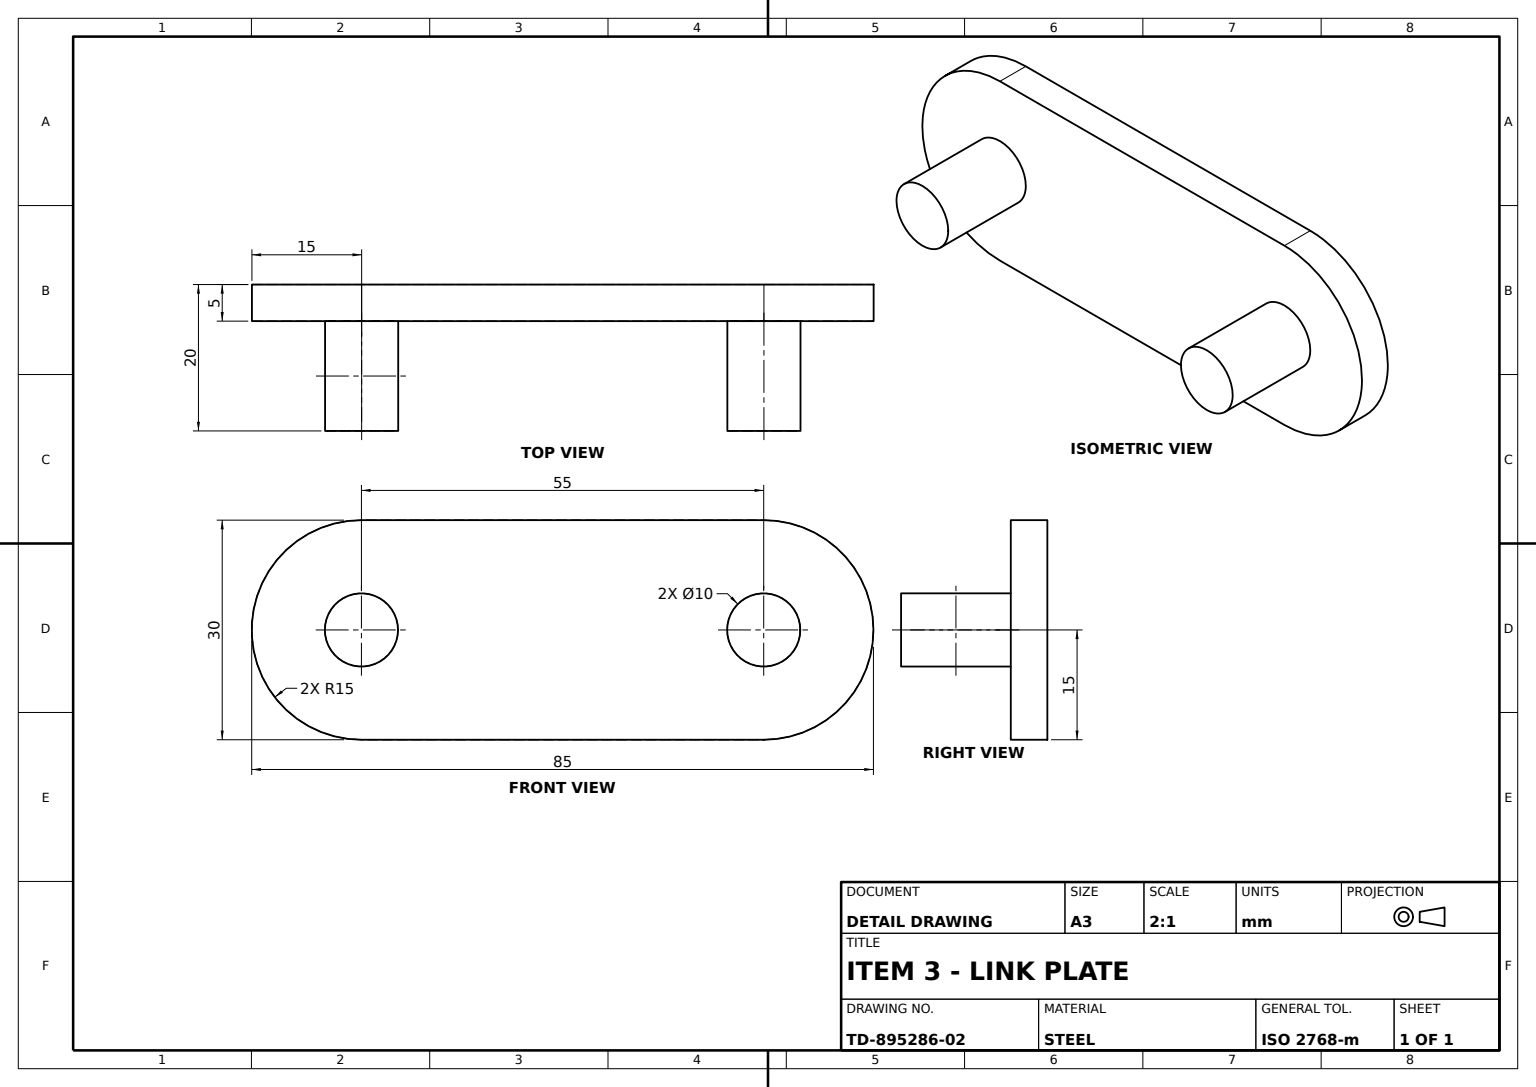
ISO-10303-21;
HEADER;
FILE_DESCRIPTION((''),'2;1');
FILE_NAME('','',(''),(''),'','','');
FILE_SCHEMA(('AUTOMOTIVE_DESIGN'));
ENDSEC;
DATA;
#1=APPLICATION_CONTEXT('');
#2=PRODUCT_CONTEXT('',#1,'mechanical');
#3=PRODUCT('','','',(#2));
#4=PRODUCT_DEFINITION_FORMATION('','',#3);
#5=PRODUCT_DEFINITION_CONTEXT('',#1,'design');
#6=PRODUCT_DEFINITION('','',#4,#5);
#7=PRODUCT_DEFINITION_SHAPE('','',#6);
#8=(LENGTH_UNIT()NAMED_UNIT(*)SI_UNIT(.MILLI.,.METRE.));
#9=(NAMED_UNIT(*)PLANE_ANGLE_UNIT()SI_UNIT($,.RADIAN.));
#10=(NAMED_UNIT(*)SI_UNIT($,.STERADIAN.)SOLID_ANGLE_UNIT());
#11=UNCERTAINTY_MEASURE_WITH_UNIT(LENGTH_MEASURE(1.E-05),#8,'distance_accuracy_value','');
#12=(GEOMETRIC_REPRESENTATION_CONTEXT(3)GLOBAL_UNCERTAINTY_ASSIGNED_CONTEXT((#11))GLOBAL_UNIT_ASSIGNED_CONTEXT((#8,#9,#10))REPRESENTATION_CONTEXT('',''));
#13=CARTESIAN_POINT('',(-22.5,0.,0.));
#14=VERTEX_POINT('',#13);
#15=CARTESIAN_POINT('',(-32.5,0.,0.));
#16=VERTEX_POINT('',#15);
#17=CARTESIAN_POINT('',(-27.5,0.,0.));
#18=DIRECTION('',(0.,0.,1.));
#19=DIRECTION('',(1.,0.,0.));
#20=AXIS2_PLACEMENT_3D('',#17,#18,#19);
#21=CIRCLE('',#20,5.);
#22=EDGE_CURVE('',#14,#16,#21,.T.);
#23=ORIENTED_EDGE('',*,*,#22,.T.);
#24=CARTESIAN_POINT('',(-32.5,0.,15.));
#25=VERTEX_POINT('',#24);
#26=DIRECTION('',(0.,0.,-1.));
#27=VECTOR('',#26,1000.);
#28=LINE('',#24,#27);
#29=EDGE_CURVE('',#25,#16,#28,.T.);
#30=ORIENTED_EDGE('',*,*,#29,.F.);
#31=CARTESIAN_POINT('',(-22.5,0.,15.));
#32=VERTEX_POINT('',#31);
#33=CARTESIAN_POINT('',(-27.5,0.,15.));
#34=AXIS2_PLACEMENT_3D('',#33,#18,#19);
#35=CIRCLE('',#34,5.);
#36=EDGE_CURVE('',#32,#25,#35,.T.);
#37=ORIENTED_EDGE('',*,*,#36,.F.);
#38=LINE('',#31,#27);
#39=EDGE_CURVE('',#32,#14,#38,.T.);
#40=ORIENTED_EDGE('',*,*,#39,.T.);
#41=EDGE_LOOP('',(#23,#30,#37,#40));
#42=FACE_OUTER_BOUND('',#41,.T.);
#43=DIRECTION('',(-1.,0.,0.));
#44=AXIS2_PLACEMENT_3D('',#33,#26,#43);
#45=CYLINDRICAL_SURFACE('',#44,5.);
#46=ADVANCED_FACE('',(#42),#45,.T.);
#47=EDGE_CURVE('',#16,#14,#21,.T.);
#48=ORIENTED_EDGE('',*,*,#47,.T.);
#49=ORIENTED_EDGE('',*,*,#39,.F.);
#50=EDGE_CURVE('',#25,#32,#35,.T.);
#51=ORIENTED_EDGE('',*,*,#50,.F.);
#52=ORIENTED_EDGE('',*,*,#29,.T.);
#53=EDGE_LOOP('',(#48,#49,#51,#52));
#54=FACE_OUTER_BOUND('',#53,.T.);
#55=ADVANCED_FACE('',(#54),#45,.T.);
#56=CARTESIAN_POINT('',(27.5,15.,-5.));
#57=VERTEX_POINT('',#56);
#58=CARTESIAN_POINT('',(27.5,15.,0.));
#59=VERTEX_POINT('',#58);
#60=VECTOR('',#18,1000.);
#61=LINE('',#56,#60);
#62=EDGE_CURVE('',#57,#59,#61,.T.);
#63=ORIENTED_EDGE('',*,*,#62,.F.);
#64=CARTESIAN_POINT('',(-27.5,15.,-5.));
#65=VERTEX_POINT('',#64);
#66=VECTOR('',#43,1000.);
#67=LINE('',#56,#66);
#68=EDGE_CURVE('',#57,#65,#67,.T.);
#69=ORIENTED_EDGE('',*,*,#68,.T.);
#70=CARTESIAN_POINT('',(-27.5,15.,0.));
#71=VERTEX_POINT('',#70);
#72=LINE('',#64,#60);
#73=EDGE_CURVE('',#65,#71,#72,.T.);
#74=ORIENTED_EDGE('',*,*,#73,.T.);
#75=LINE('',#58,#66);
#76=EDGE_CURVE('',#59,#71,#75,.T.);
#77=ORIENTED_EDGE('',*,*,#76,.F.);
#78=EDGE_LOOP('',(#63,#69,#74,#77));
#79=FACE_OUTER_BOUND('',#78,.T.);
#80=DIRECTION('',(0.,1.,0.));
#81=AXIS2_PLACEMENT_3D('',#56,#80,#43);
#82=PLANE('',#81);
#83=ADVANCED_FACE('',(#79),#82,.T.);
#84=CARTESIAN_POINT('',(32.5,0.,15.));
#85=VERTEX_POINT('',#84);
#86=CARTESIAN_POINT('',(22.5,0.,15.));
#87=VERTEX_POINT('',#86);
#88=CARTESIAN_POINT('',(27.5,0.,15.));
#89=AXIS2_PLACEMENT_3D('',#88,#18,#19);
#90=CIRCLE('',#89,5.);
#91=EDGE_CURVE('',#85,#87,#90,.T.);
#92=ORIENTED_EDGE('',*,*,#91,.T.);
#93=EDGE_CURVE('',#87,#85,#90,.T.);
#94=ORIENTED_EDGE('',*,*,#93,.T.);
#95=EDGE_LOOP('',(#92,#94));
#96=FACE_OUTER_BOUND('',#95,.T.);
#97=CARTESIAN_POINT('',(0.,0.,15.));
#98=AXIS2_PLACEMENT_3D('',#97,#18,#19);
#99=PLANE('',#98);
#100=ADVANCED_FACE('',(#96),#99,.T.);
#101=CARTESIAN_POINT('',(-27.5,-15.,-5.));
#102=VERTEX_POINT('',#101);
#103=CARTESIAN_POINT('',(-27.5,0.,-5.));
#104=AXIS2_PLACEMENT_3D('',#103,#18,#19);
#105=CIRCLE('',#104,15.);
#106=EDGE_CURVE('',#65,#102,#105,.T.);
#107=ORIENTED_EDGE('',*,*,#106,.T.);
#108=CARTESIAN_POINT('',(-27.5,-15.,0.));
#109=VERTEX_POINT('',#108);
#110=LINE('',#101,#60);
#111=EDGE_CURVE('',#102,#109,#110,.T.);
#112=ORIENTED_EDGE('',*,*,#111,.T.);
#113=CIRCLE('',#20,15.);
#114=EDGE_CURVE('',#71,#109,#113,.T.);
#115=ORIENTED_EDGE('',*,*,#114,.F.);
#116=ORIENTED_EDGE('',*,*,#73,.F.);
#117=EDGE_LOOP('',(#107,#112,#115,#116));
#118=FACE_OUTER_BOUND('',#117,.T.);
#119=CYLINDRICAL_SURFACE('',#104,15.);
#120=ADVANCED_FACE('',(#118),#119,.T.);
#121=ORIENTED_EDGE('',*,*,#91,.F.);
#122=CARTESIAN_POINT('',(32.5,0.,0.));
#123=VERTEX_POINT('',#122);
#124=LINE('',#84,#27);
#125=EDGE_CURVE('',#85,#123,#124,.T.);
#126=ORIENTED_EDGE('',*,*,#125,.T.);
#127=CARTESIAN_POINT('',(22.5,0.,0.));
#128=VERTEX_POINT('',#127);
#129=CARTESIAN_POINT('',(27.5,0.,0.));
#130=AXIS2_PLACEMENT_3D('',#129,#18,#19);
#131=CIRCLE('',#130,5.);
#132=EDGE_CURVE('',#123,#128,#131,.T.);
#133=ORIENTED_EDGE('',*,*,#132,.T.);
#134=LINE('',#86,#27);
#135=EDGE_CURVE('',#87,#128,#134,.T.);
#136=ORIENTED_EDGE('',*,*,#135,.F.);
#137=EDGE_LOOP('',(#121,#126,#133,#136));
#138=FACE_OUTER_BOUND('',#137,.T.);
#139=AXIS2_PLACEMENT_3D('',#88,#26,#43);
#140=CYLINDRICAL_SURFACE('',#139,5.);
#141=ADVANCED_FACE('',(#138),#140,.T.);
#142=CARTESIAN_POINT('',(42.5,0.,0.));
#143=VERTEX_POINT('',#142);
#144=CIRCLE('',#130,15.);
#145=EDGE_CURVE('',#143,#59,#144,.T.);
#146=ORIENTED_EDGE('',*,*,#145,.F.);
#147=CARTESIAN_POINT('',(42.5,0.,-5.));
#148=VERTEX_POINT('',#147);
#149=LINE('',#147,#60);
#150=EDGE_CURVE('',#148,#143,#149,.T.);
#151=ORIENTED_EDGE('',*,*,#150,.F.);
#152=CARTESIAN_POINT('',(27.5,0.,-5.));
#153=AXIS2_PLACEMENT_3D('',#152,#18,#19);
#154=CIRCLE('',#153,15.);
#155=EDGE_CURVE('',#148,#57,#154,.T.);
#156=ORIENTED_EDGE('',*,*,#155,.T.);
#157=ORIENTED_EDGE('',*,*,#62,.T.);
#158=EDGE_LOOP('',(#146,#151,#156,#157));
#159=FACE_OUTER_BOUND('',#158,.T.);
#160=CYLINDRICAL_SURFACE('',#153,15.);
#161=ADVANCED_FACE('',(#159),#160,.T.);
#162=ORIENTED_EDGE('',*,*,#22,.F.);
#163=ORIENTED_EDGE('',*,*,#47,.F.);
#164=EDGE_LOOP('',(#162,#163));
#165=FACE_BOUND('',#164,.T.);
#166=ORIENTED_EDGE('',*,*,#145,.T.);
#167=ORIENTED_EDGE('',*,*,#76,.T.);
#168=ORIENTED_EDGE('',*,*,#114,.T.);
#169=CARTESIAN_POINT('',(27.5,-15.,0.));
#170=VERTEX_POINT('',#169);
#171=LINE('',#169,#66);
#172=EDGE_CURVE('',#170,#109,#171,.T.);
#173=ORIENTED_EDGE('',*,*,#172,.F.);
#174=EDGE_CURVE('',#170,#143,#144,.T.);
#175=ORIENTED_EDGE('',*,*,#174,.T.);
#176=EDGE_LOOP('',(#166,#167,#168,#173,#175));
#177=FACE_OUTER_BOUND('',#176,.T.);
#178=EDGE_CURVE('',#128,#123,#131,.T.);
#179=ORIENTED_EDGE('',*,*,#178,.F.);
#180=ORIENTED_EDGE('',*,*,#132,.F.);
#181=EDGE_LOOP('',(#179,#180));
#182=FACE_BOUND('',#181,.T.);
#183=PLANE('',#130);
#184=ADVANCED_FACE('',(#165,#177,#182),#183,.T.);
#185=ORIENTED_EDGE('',*,*,#93,.F.);
#186=ORIENTED_EDGE('',*,*,#135,.T.);
#187=ORIENTED_EDGE('',*,*,#178,.T.);
#188=ORIENTED_EDGE('',*,*,#125,.F.);
#189=EDGE_LOOP('',(#185,#186,#187,#188));
#190=FACE_OUTER_BOUND('',#189,.T.);
#191=ADVANCED_FACE('',(#190),#140,.T.);
#192=CARTESIAN_POINT('',(27.5,-15.,-5.));
#193=VERTEX_POINT('',#192);
#194=EDGE_CURVE('',#193,#148,#154,.T.);
#195=ORIENTED_EDGE('',*,*,#194,.F.);
#196=LINE('',#192,#66);
#197=EDGE_CURVE('',#193,#102,#196,.T.);
#198=ORIENTED_EDGE('',*,*,#197,.T.);
#199=ORIENTED_EDGE('',*,*,#106,.F.);
#200=ORIENTED_EDGE('',*,*,#68,.F.);
#201=ORIENTED_EDGE('',*,*,#155,.F.);
#202=EDGE_LOOP('',(#195,#198,#199,#200,#201));
#203=FACE_OUTER_BOUND('',#202,.T.);
#204=PLANE('',#153);
#205=ADVANCED_FACE('',(#203),#204,.F.);
#206=ORIENTED_EDGE('',*,*,#194,.T.);
#207=ORIENTED_EDGE('',*,*,#150,.T.);
#208=ORIENTED_EDGE('',*,*,#174,.F.);
#209=LINE('',#192,#60);
#210=EDGE_CURVE('',#193,#170,#209,.T.);
#211=ORIENTED_EDGE('',*,*,#210,.F.);
#212=EDGE_LOOP('',(#206,#207,#208,#211));
#213=FACE_OUTER_BOUND('',#212,.T.);
#214=ADVANCED_FACE('',(#213),#160,.T.);
#215=ORIENTED_EDGE('',*,*,#36,.T.);
#216=ORIENTED_EDGE('',*,*,#50,.T.);
#217=EDGE_LOOP('',(#215,#216));
#218=FACE_OUTER_BOUND('',#217,.T.);
#219=ADVANCED_FACE('',(#218),#99,.T.);
#220=ORIENTED_EDGE('',*,*,#197,.F.);
#221=ORIENTED_EDGE('',*,*,#210,.T.);
#222=ORIENTED_EDGE('',*,*,#172,.T.);
#223=ORIENTED_EDGE('',*,*,#111,.F.);
#224=EDGE_LOOP('',(#220,#221,#222,#223));
#225=FACE_OUTER_BOUND('',#224,.T.);
#226=AXIS2_PLACEMENT_3D('',#192,#80,#43);
#227=PLANE('',#226);
#228=ADVANCED_FACE('',(#225),#227,.F.);
#229=CLOSED_SHELL('',(#46,#55,#83,#100,#120,#141,#161,#184,#191,#205,#214,#219,#228));
#230=MANIFOLD_SOLID_BREP('',#229);
#231=ADVANCED_BREP_SHAPE_REPRESENTATION('',(#230),#12);
#232=SHAPE_DEFINITION_REPRESENTATION(#7,#231);
ENDSEC;
END-ISO-10303-21;
